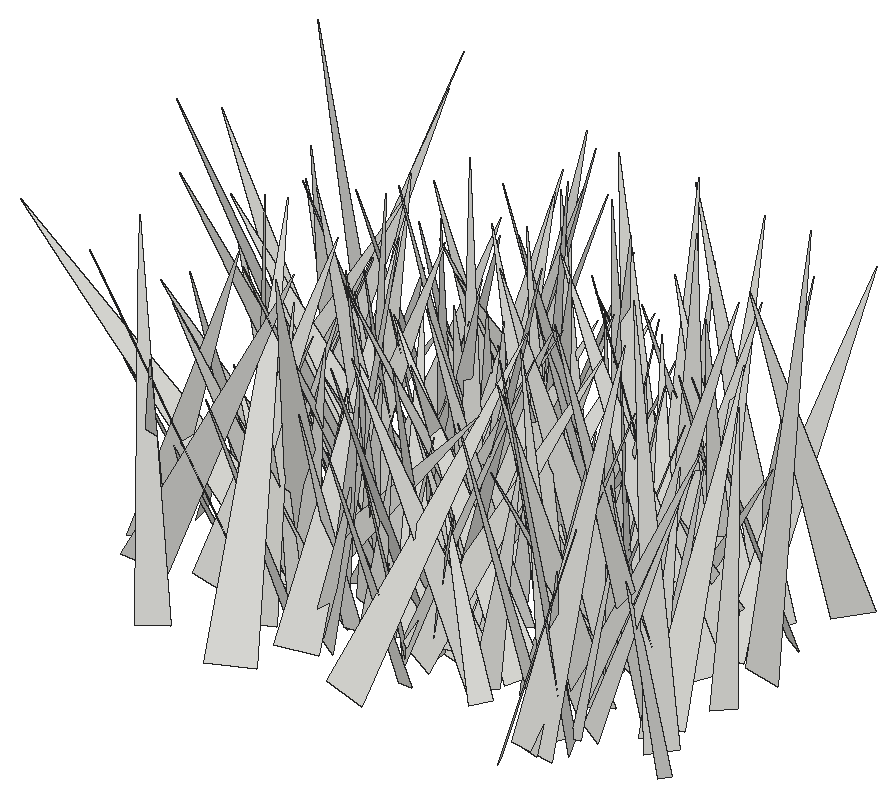
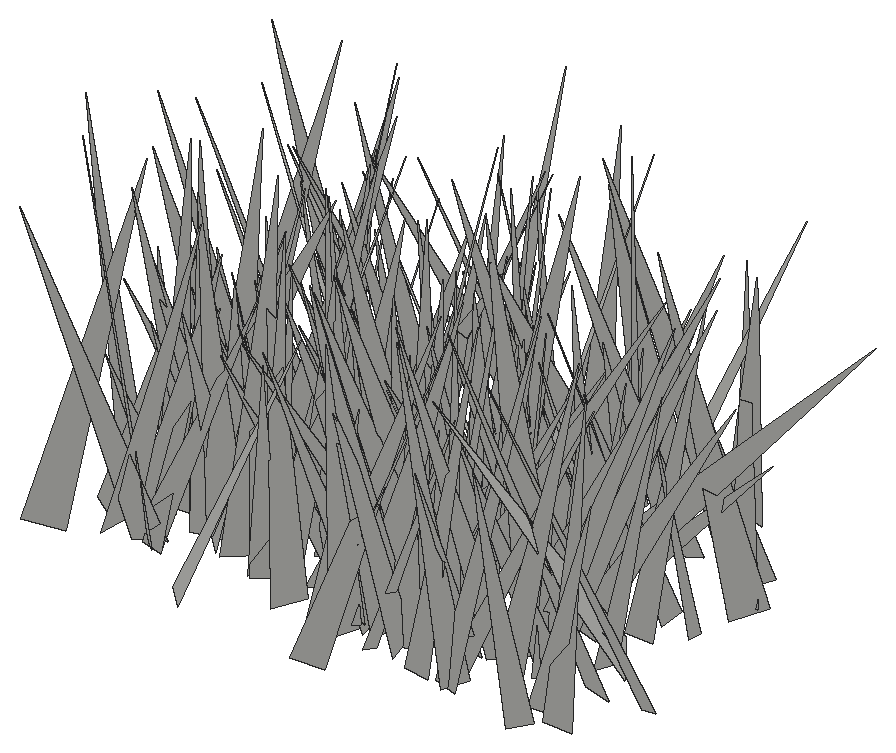
# SketchUp Ruby script. Lengths in inches.
U = 1.inch
M = Sketchup.active_model
def pt(a) = Geom::Point3d.new(a.map { |v| v * U })
def face(e, loops, mat)
  f = e.add_face(loops[0].map { |a| pt(a) })
  loops[1..].each { |l| e.add_face(l.map { |a| pt(a) }).erase! }
  f.material = f.back_material = mat if mat
  f
end
# faces: each face lists its corners as indices into pts; further lists are holes
def faces(e, pts, list, mat = nil) = list.each { |f| face(e, (f[0].is_a?(Array) ? f : [f]).map { |l| l.map { |i| pts[i] } }, mat) }
# xy, xz, yz: faces in a plane at the given z, y or x. An outline is a flat list of corners, or four numbers for a rectangle; further outlines are holes
def ring(l) = l.size == 4 ? [[l[0], l[1]], [l[2], l[1]], [l[2], l[3]], [l[0], l[3]]] : l.each_slice(2).to_a
def flat(e, list, mat, &to3) = list.each { |f| face(e, (f[0].is_a?(Array) ? f : [f]).map { |l| ring(l).map { |u, v| to3.(u, v) } }, mat) }
def xy(e, z, list, mat = nil) = flat(e, list, mat) { |x, y| [x, y, z] }
def xz(e, y, list, mat = nil) = flat(e, list, mat) { |x, z| [x, y, z] }
def yz(e, x, list, mat = nil) = flat(e, list, mat) { |y, z| [x, y, z] }
def lines(e, pts, list) = list.each { |a, b| e.add_line(pt(pts[a]), pt(pts[b])) }
# prism: a flat outline (further loops are holes) pulled along v
def prism(e, loops, v, mat = nil)
  f = face(e, loops, mat); d = Geom::Vector3d.new(v.map { |x| x * U })
  f.pushpull(f.normal.samedirection?(d) ? d.length : -d.length)
end
def box(e, o, s, mat = nil) = prism(e, [[o, [o[0] + s[0], o[1], o[2]], [o[0] + s[0], o[1] + s[1], o[2]], [o[0], o[1] + s[1], o[2]]]], [0, 0, s[2]], mat)
def at(x, y, z, deg = 0) = Geom::Transformation.translation(pt([x, y, z])) * Geom::Transformation.rotation(ORIGIN, Z_AXIS, deg.degrees)
def axes(o, x, y, z) = Geom::Transformation.new([*x, 0, *y, 0, *z, 0, *pt(o).to_a, 1])
def part(name) = M.definitions.add(name)
# library, detail: a bought-in or finely detailed component or shape, given as its bounding box
def library(name, o, s) = part(name).tap { |d| box(d.entities, o, s) }
def detail(e, o, s) = box(e.add_group.entities, o, s)
def put(e, d, t, mat = nil) = e.add_instance(d, t).tap { |i| i.material = mat if mat }
def group(e, t, mat = nil) = e.add_group.tap { |g| g.transformation = t; g.material = mat if mat }.entities
root = M.entities
c1 = part("fur_instance\#9")
p = [[0.8125,0,1.79],[0.67,-0.02,1.48],[0,-0.11,0],[0,0.11,0]]
faces(c1.entities,p,[[0,1,2,3]])
put(root,c1,axes([493.16,72.27,-21.86],[-2.05485,-3.90462,0.97999],[-3.96047,1.76344,-1.27819],[-0.72186,1.43981,4.22312]))
put(root,c1,axes([484.04,69.875,-21.66],[-0.66678,7.09806,0.59701],[6.83624,0.46921,2.05647],[-2.00116,-0.76214,6.82627]))
put(root,c1,axes([488.25,72.6,-21.86],[-2.14589,-4.13922,0.79032],[-4.13009,1.88974,-1.31675],[-0.83673,1.28775,4.4726]))
put(root,c1,axes([490.875,75.99,-21.86],[-2.64275,-7.72517,0.10148],[-7.35563,2.5487,2.46402],[2.36287,-0.70608,7.78402]))
put(root,c1,axes([485.3,73.87,-21.86],[-4.92734,-5.46841,0.2776],[-5.45988,4.87887,-0.80338],[-0.41255,0.74316,7.31688]))
put(root,c1,axes([500.3,72.47,-21.86],[-6.28358,-3.49392,1.76213],[-3.72095,6.36668,-0.64478],[1.21124,1.43309,7.16066]))
put(root,c1,axes([480.18,74.73,-21.86],[0.06322,-6.05576,0.15688],[-5.74231,-0.00994,1.93043],[1.92942,0.16885,5.74018]))
put(root,c1,axes([498.93,70.22,-21.86],[5.00084,3.55671,0.83126],[3.26277,-4.98345,1.69387],[-1.6418,0.92989,5.89825]))
put(root,c1,axes([487.64,69.6,-21.86],[-4.43994,6.98412,0.3729],[6.94517,4.45476,-0.74146],[0.82561,0.08476,8.24265]))
put(root,c1,axes([498.52,73.41,-21.86],[3.38817,-1.89067,0.4047],[-1.85762,-3.4096,-0.37677],[-0.53632,-0.13453,3.86165]))
put(root,c1,axes([499.5,71.25,-21.86],[1.47589,3.3854,0.35503],[3.34161,-1.51469,0.55196],[-0.64858,-0.1002,3.65165]))
put(root,c1,axes([499.47,71.32,-21.86],[0.16612,7.76506,1.97129],[7.95416,0.07536,-0.96713],[0.95574,-1.97685,7.70638]))
put(root,c1,axes([491.76,74.06,-21.86],[-3.13954,-2.86345,1.03549],[-2.74612,3.30524,0.81394],[1.31545,0.06589,4.17056]))
put(root,c1,axes([480.91,73.3,-21.86],[4.47531,-6.51665,1.20055],[-6.35255,-3.80729,3.0143],[1.88498,2.64087,7.30815]))
put(root,c1,axes([495.11,74.09,-21.86],[-6.35837,1.48,1.02188],[1.69793,6.17763,1.61781],[0.593,-1.81932,6.3247]))
put(root,c1,axes([488.86,72.93,-21.86],[3.38987,-1.12165,1.00676],[-1.27426,-3.45624,0.43994],[-0.80492,0.7478,3.54341]))
put(root,c1,axes([491.9,70.51,-21.86],[0.36828,7.38641,0.21711],[7.15433,-0.30198,-1.86176],[1.84979,-0.30261,7.15741]))
put(root,c1,axes([488.36,74.56,-21.86],[-1.36067,-5.7583,1.83351],[-5.61411,1.9,1.80082],[2.23642,1.26617,5.63617]))
put(root,c1,axes([495.96,72.91,-21.86],[-2.71204,2.5664,0.21286],[2.56651,2.66825,0.52947],[-0.21147,-0.53003,3.69611]))
put(root,c1,axes([499.19,75.12,-21.86],[1.49882,-6.76146,1.59023],[-6.75855,-1.79498,-1.262],[-1.60255,1.24632,6.80963]))
put(root,c1,axes([492.45,74.44,-21.86],[3.23905,1.92957,1.10614],[2.22288,-2.8741,-1.49551],[-0.07469,-1.85863,3.46094]))
put(root,c1,axes([490.24,74.02,-21.86],[2.26375,-3.28304,0.92587],[-3.40814,-2.22313,0.4499],[-0.14199,1.01955,3.96238]))
put(root,c1,axes([486.47,75.3,-21.66],[1.14957,-5.99203,1.40359],[-5.68779,-1.57972,-2.08556],[-2.35023,0.89221,5.73379]))
put(root,c1,axes([489.35,74.21,-21.86],[-0.77658,-4.10323,1.17838],[-4.23531,0.59015,-0.73621],[-0.53592,1.28194,4.11067]))
put(root,c1,axes([497.34,74.18,-21.86],[-4.90258,-2.23132,0.87524],[-2.28191,4.95484,-0.15015],[0.73329,0.50088,5.38438]))
put(root,c1,axes([499.65,72.49,-21.86],[-6.80477,1.06742,0.77743],[0.9228,6.76292,-1.20833],[0.94457,1.0827,6.78117]))
put(root,c1,axes([491.02,76.2,-21.66],[-2.08812,-6.42397,1.05341],[-6.15561,2.30841,1.87538],[2.11792,0.37569,6.48927]))
put(root,c1,axes([486.1,75.07,-21.86],[5.26826,5.58359,0.80335],[4.69893,-3.73546,-4.8521],[3.1212,-3.80083,5.9488]))
put(root,c1,axes([485.46,73.93,-21.86],[4.5767,5.68819,3.18986],[6.17982,-5.02762,0.09872],[-2.08339,-2.41752,7.30013]))
put(root,c1,axes([495.46,73.79,-21.86],[3.51253,-2.51047,1.78394],[-2.89575,-3.6135,0.61652],[-1.0486,1.56939,4.2732]))
put(root,c1,axes([485.29,77.09,-21.86],[6.31463,-5.10403,0.36931],[-4.97216,-6.25818,-1.47472],[-1.21044,-0.91981,7.98441]))
put(root,c1,axes([485.09,75.43,-21.86],[3.48904,-1.79502,0.75996],[-1.60226,-3.52839,-0.97792],[-1.11014,-0.54905,3.7999]))
put(root,c1,axes([504.12,72.79,-21.86],[-5.07583,-0.99149,0.0646],[-0.93064,4.62637,-2.11704],[-0.34804,2.08923,4.7186]))
put(root,c1,axes([490.82,74.28,-21.86],[2.69077,3.3772,1.27263],[3.60609,-2.57991,-0.77814],[-0.14558,-1.48455,4.24737]))
put(root,c1,axes([500.26,73.55,-21.86],[2.30047,4.4169,0.81433],[4.47004,-2.16262,-0.89782],[0.43686,-1.13065,4.89848]))
put(root,c1,axes([498.04,77.22,-21.86],[-4.51609,-3.87484,0.43498],[-3.47065,4.29803,2.25393],[1.77713,-1.453,5.5072]))
put(root,c1,axes([502,75.12,-21.66],[-1.47229,-7.46087,2.3597],[-7.72207,0.99683,-1.66627],[-1.2659,2.59656,7.41996]))
put(root,c1,axes([496.22,74.83,-21.66],[5.98331,3.57339,0.75673],[3.63565,-5.68637,-1.89446],[0.35186,-2.00943,6.70672]))
put(root,c1,axes([500.3,72.66,-21.66],[1.53322,3.39,0.04746],[3.12816,-1.43461,1.41479],[-1.30727,0.54307,3.44111]))
put(root,c1,axes([489.37,72.72,-21.86],[4.31579,6.0344,1.65644],[5.97789,-4.5707,1.07586],[-1.85004,-0.69181,7.34048]))
put(root,c1,axes([485.4,75.46,-21.86],[0.28978,-3.77503,0.68612],[-3.83038,-0.24462,0.27184],[0.22308,0.70349,3.77636]))
put(root,c1,axes([486.96,72.23,-21.66],[-5.33411,1.7362,0.45715],[1.45522,5.02033,-2.08679],[1.05153,1.85957,5.20696]))
put(root,c1,axes([498.81,74.43,-21.66],[3.86219,5.07234,0.99731],[5.04282,-3.42294,-2.11973],[1.1372,-2.04809,6.01264]))
put(root,c1,axes([490.53,74.68,-21.86],[5.38161,2.47127,3.67462],[2.66712,-6.4254,0.41515],[-3.53503,-1.08568,5.90733]))
put(root,c1,axes([483.8,73.36,-21.66],[-0.17372,7.00266,1.70424],[6.95108,0.61311,-1.81067],[1.90374,-1.5996,6.76675]))
put(root,c1,axes([484.52,74.32,-21.66],[-3.03964,-3.22245,0.08473],[-2.53096,2.3136,-2.80576],[-1.9964,1.97328,3.42802]))
put(root,c1,axes([479.75,74.93,-21.86],[5.60342,-3.67276,1.04707],[-3.81273,-5.48708,1.15708],[-0.22057,1.54484,6.59914]))
put(root,c1,axes([491.8,73.81,-21.86],[4.90909,4.36789,0.50992],[4.39704,-4.86378,-0.66882],[0.06695,-0.83837,6.53684]))
put(root,c1,axes([487.25,73.77,-21.86],[-4.58169,-0.00231,0.33908],[-0.10273,4.38765,-1.35823],[0.32316,1.36211,4.37574]))
put(root,c1,axes([485.61,75.91,-21.86],[-5.86481,5.71927,0.12396],[4.62698,4.63811,4.91939],[-3.36399,-3.59156,6.55024]))
put(root,c1,axes([487.5,78.6,-21.66],[-5.6893,-5.57398,0.54513],[-5.22917,5.56506,2.3282],[2.00554,-1.30211,7.61688]))
put(root,c1,axes([492.47,73.71,-21.66],[1.86343,6.88556,0.79652],[6.51007,-1.45535,-2.64927],[2.37997,-1.41024,6.62304]))
put(root,c1,axes([496.75,76.26,-21.86],[4.53456,1.85789,3.16607],[2.55783,-5.20835,-0.60709],[-2.63311,-1.85992,4.86266]))
put(root,c1,axes([485.8,75.9375,-21.86],[0.23103,-4.99246,1.62863],[-5.17408,0.0623,0.92493],[0.89778,1.64376,4.91147]))
put(root,c1,axes([488.94,71.58,-21.66],[-6.13074,4.86156,0.06985],[4.48302,5.69573,-2.94734],[1.88206,2.26926,7.24803]))
put(root,c1,axes([490.07,75.71,-21.66],[-2.15609,-3.98258,0.83043],[-3.73233,1.56246,-2.1972],[-1.61872,1.70208,3.96005]))
put(root,c1,axes([492.79,74.95,-21.86],[7.58691,1.58366,1.76713],[1.48707,-7.78642,0.59349],[-1.84915,0.23586,7.72768]))
put(root,c1,axes([496.28,74.88,-21.66],[-3.37764,5.82202,0.02709],[5.22944,3.02002,2.9728],[-2.55923,-1.51283,6.03878]))
put(root,c1,axes([485.65,75.42,-21.86],[-2.38468,3.13652,0.12042],[3.02513,2.25628,1.13874],[-0.83714,-0.7813,3.77197]))
put(root,c1,axes([493.81,78.08,-21.86],[-6.74137,-3.47517,0.05647],[-3.44773,6.70195,0.85032],[0.43951,-0.73012,7.53656]))
put(root,c1,axes([484.62,74.375,-21.86],[3.35621,4.76804,0.53975],[4.75729,-3.3924,0.38655],[-0.62744,-0.21695,5.81798]))
put(root,c1,axes([503.14,73.84,-21.66],[-7.7657,1.30292,0.44128],[1.14319,7.51969,-2.08465],[0.76515,1.98873,7.59328]))
put(root,c1,axes([492.96,74.78,-21.86],[0.42201,3.83383,0.13948],[3.79822,-0.3978,-0.55775],[0.53966,-0.19825,3.81644]))
put(root,c1,axes([486.6,74.625,-21.86],[3.67967,2.76321,1.03507],[2.46473,-3.78797,1.35021],[-1.62229,0.51247,4.39911]))
put(root,c1,axes([495.53,77.25,-21.86],[-0.9776,-5.25666,1.94415],[-5.10339,1.65068,1.89699],[2.31681,1.41798,4.99896]))
put(root,c1,axes([493.32,74.91,-21.66],[-2.78361,3.37072,1.19614],[3.02117,3.0272,-1.49988],[1.91443,0.12385,4.10617]))
put(root,c1,axes([502.02,74.66,-21.86],[-4.30895,1.90574,0.59057],[1.67064,4.21479,-1.41144],[1.09067,1.07302,4.49519]))
put(root,c1,axes([490.04,77.36,-21.86],[-0.65259,-3.58567,0.77528],[-3.62638,0.74954,0.41412],[0.55447,0.682,3.62097]))
put(root,c1,axes([481.67,78.54,-21.86],[-0.57876,-6.04691,0.53315],[-6.05695,0.61084,0.35302],[0.40347,0.49606,6.06428]))
put(root,c1,axes([489.11,77.16,-21.66],[1.07794,-7.21694,3.00432],[-7.53412,-1.768,-1.54384],[-2.08502,2.65746,7.13181]))
put(root,c1,axes([491.26,74.95,-21.86],[-1.93628,5.55,0.46539],[5.55779,1.89356,0.54185],[-0.36056,-0.61659,5.85304]))
put(root,c1,axes([488.66,75.8,-21.86],[3.17531,6.56755,2.54139],[6.79761,-3.58673,0.77578],[-1.83954,-1.91744,7.25351]))
put(root,c1,axes([487.5625,78.01,-21.86],[2.55514,-3.36467,0.69917],[-3.31318,-2.64324,-0.61213],[-0.91251,0.1757,4.18031]))
put(root,c1,axes([486.22,76.21,-21.66],[3.6811,-6.05089,2.6185],[-6.53456,-2.94932,2.37094],[0.87715,3.42178,6.67401]))
put(root,c1,axes([492.45,77.01,-21.86],[-3.8674,0.14725,0.40736],[0.1724,3.88071,0.23399],[0.39736,-0.25058,3.86312]))
put(root,c1,axes([497.97,74.56,-21.86],[-8.22184,1.12863,0.67504],[0.91948,7.98903,-2.15825],[0.94024,2.05661,8.01339]))
put(root,c1,axes([480.26,77.26,-21.86],[3.62066,0.28745,0.41277],[0.34104,-3.60783,-0.479],[-0.36973,-0.51296,3.60033]))
put(root,c1,axes([493.85,77.6,-21.66],[-0.12405,-5.8754,2.10648],[-6.00776,-0.4589,-1.63376],[-1.69244,2.05962,5.64504]))
put(root,c1,axes([487.54,79.42,-21.66],[-3.32814,-6.39102,1.50803],[-6.07577,3.63841,2.01068],[2.49085,0.3356,6.91945]))
put(root,c1,axes([487.49,76.84,-21.86],[4.11337,-1.35782,0.42666],[-1.42017,-4.00175,0.95638],[-0.09392,1.04301,4.22479]))
put(root,c1,axes([487.9,77.13,-21.86],[-3.35833,-3.2337,1.73378],[-3.57177,3.41915,-0.54142],[0.83981,1.61055,4.63056]))
put(root,c1,axes([490.22,80.32,-21.66],[5.08436,-3.96797,0.13679],[-3.71243,-4.83007,-2.12193],[-1.40762,-1.5937,6.0904]))
put(root,c1,axes([481.64,76.8,-21.86],[4.44559,-0.41699,0.42413],[-0.48383,-4.39553,0.74982],[-0.34594,0.78895,4.4017]))
put(root,c1,axes([497.54,78.56,-21.66],[2.58278,-6.81445,2.81399],[-6.72051,-3.40212,-2.07037],[-3.03151,1.73634,6.98721]))
put(root,c1,axes([502.14,75.22,-21.66],[-4.09876,5.0884,1.14662],[4.86258,4.25523,-1.50159],[1.8873,0.0873,6.359]))
put(root,c1,axes([488.97,77.59,-21.86],[-5.40914,1.11965,1.3835],[1.23539,5.5484,0.3398],[1.28121,-0.62292,5.51334]))
put(root,c1,axes([483.52,79.38,-21.86],[0.83306,-5.07313,1.39633],[-4.3947,-1.44829,-2.63999],[-2.89363,0.73905,4.41148]))
put(root,c1,axes([495.43,79.36,-21.86],[1.75124,-3.26229,0.83742],[-3.12175,-1.92651,-0.97669],[-1.26432,0.23809,3.57148]))
put(root,c1,axes([488.97,79.05,-21.86],[2.93254,-6.52755,1.0505],[-6.19008,-2.30697,2.94501],[2.32281,2.09313,6.52193]))
put(root,c1,axes([488.57,79.72,-21.86],[-0.29394,-4.28793,0.2812],[-4.0742,0.18848,-1.38464],[-1.36614,0.36048,4.06885]))
put(root,c1,axes([488.78,80.11,-21.86],[-3.34858,-4.98605,1.16696],[-4.83329,3.53804,1.24784],[1.69169,0.23891,5.87509]))
put(root,c1,axes([491.71,79.5,-21.86],[-7.3935,-3.44968,1.78048],[-3.41196,7.60131,0.55924],[1.85173,0.23234,8.13949]))
put(root,c1,axes([500.63,76.88,-21.66],[-3.9364,0.91485,1.26316],[0.41585,3.92071,-1.54367],[1.50319,1.31107,3.73488]))
put(root,c1,axes([493.23,80.95,-21.66],[5.19652,-2.78136,0.42044],[-2.54268,-5.02221,-1.79688],[-1.20313,-1.39929,5.61347]))
put(root,c1,axes([498.26,77.73,-21.66],[2.40948,7.1196,1.80641],[7.28749,-2.07931,-1.52526],[0.91887,-2.17835,7.35989]))
put(root,c1,axes([488.34,79.875,-21.86],[-7.10232,2.48969,0.17848],[2.39972,6.66255,2.55443],[-0.68683,-2.46683,7.07929]))
put(root,c1,axes([484.66,79.36,-21.86],[1.69765,-3.69471,0.41656],[-3.54176,-1.46758,1.41724],[1.13153,0.9496,3.81108]))
put(root,c1,axes([492.5,76.81,-21.86],[1.13757,8.04859,1.54719],[7.76789,-1.55698,2.3882],[-2.61411,-1.12413,7.76984]))
put(root,c1,axes([489.38,77.33,-21.86],[-2.89965,3.32427,1.06428],[2.78447,3.03733,-1.90073],[2.1048,0.5615,3.98069]))
put(root,c1,axes([502.71,77.75,-21.86],[-4.9436,1.78617,0.77223],[1.56135,4.89918,-1.33648],[1.16143,1.01666,5.08364]))
put(root,c1,axes([501.0625,78.72,-21.66],[-3.57057,6.8988,1.02898],[6.50769,2.8788,3.28081],[-2.51043,-2.34953,7.04122]))
put(root,c1,axes([483.25,81.69,-21.66],[0.03934,-7.1777,0.79174],[-6.87762,-0.27857,-2.18369],[-2.20103,0.74216,6.83757]))
put(root,c1,axes([498.2,77.43,-21.86],[-6.18556,-0.57175,1.0735],[-0.94708,5.75521,-2.39186],[0.76312,2.5082,5.73298]))
put(root,c1,axes([484.83,80.61,-21.66],[-3.02685,-7.70536,1.30124],[-7.48247,2.45538,-2.86554],[-2.25353,2.19686,7.76679]))
put(root,c1,axes([496.55,80.3,-21.86],[-4.3896,-2.50757,2.34029],[-2.3133,4.97071,0.98703],[2.5325,0.19407,4.95805]))
put(root,c1,axes([494.53,79.03,-21.86],[-6.29408,3.56033,1.19684],[3.6784,6.31519,0.55815],[0.76008,-1.07993,7.20971]))
put(root,c1,axes([495.375,79.7,-21.86],[0.04539,-4.24616,1.86431],[-4.44886,0.48634,1.21602],[1.30888,1.80033,4.06857]))
put(root,c1,axes([487.52,79.37,-21.86],[5.08569,0.11573,0.95874],[0.07501,-5.17107,0.22632],[-0.96278,0.20845,5.08197]))
put(root,c1,axes([485.05,79.7,-21.86],[-2.73382,6.12597,3.74599],[6.6709,3.64992,-1.10045],[2.6569,-2.86083,6.61742]))
put(root,c1,axes([488.39,81.15,-21.86],[-3.41179,-1.77285,0.16017],[-1.67154,3.30984,1.02951],[0.61205,-0.84317,3.70451]))
put(root,c1,axes([487.1,81.73,-21.66],[1.41766,-6.83451,0.48866],[-6.53171,-1.19719,2.20513],[2.07029,0.90294,6.62252]))
put(root,c1,axes([487.97,79.57,-21.66],[4.83025,3.81866,0.07193],[3.65702,-4.5907,-1.86288],[1.10161,-1.50398,5.86882]))
put(root,c1,axes([489.02,81.15,-21.86],[3.24454,-4.71501,1.03025],[-4.7617,-3.32972,-0.24278],[-0.78672,0.70811,5.71834]))
put(root,c1,axes([481.32,80.81,-21.86],[-5.12264,0.34016,1.65759],[0.60899,5.30124,0.79415],[1.57874,-0.94118,5.07212]))
put(root,c1,axes([496.36,78.82,-21.86],[3.89284,1.77366,0.49192],[1.64576,-3.86945,0.92782],[-0.82421,0.65077,4.17603]))
put(root,c1,axes([496.83,79.75,-21.86],[-7.44301,-3.63877,0.95843],[-3.76282,7.20814,-1.85509],[0.01898,2.08796,8.0745]))
put(root,c1,axes([490.09,80.75,-21.86],[4.42383,-2.92058,1.2942],[-2.99041,-4.56361,-0.07677],[-1.12348,0.64702,5.30039]))
put(root,c1,axes([492.28,79.63,-21.86],[-1.46329,-3.87448,2.4887],[-4.52721,1.6881,-0.03379],[0.84239,2.34204,4.14146]))
put(root,c1,axes([500.63,82.02,-21.86],[2.63611,-2.6678,0.56163],[-2.26437,-2.5776,-1.61563],[-1.51829,-0.78771,3.38467]))
put(root,c1,axes([498.41,79.66,-21.66],[4.05513,-1.76427,0.28786],[-1.75227,-3.78191,1.50543],[0.35366,1.49134,4.15818]))
put(root,c1,axes([491.34,78.47,-21.86],[-5.55671,4.70477,2.20019],[4.40361,5.97611,-1.65743],[2.7539,-0.06297,7.08977]))
put(root,c1,axes([495.97,80,-21.86],[4.05853,2.67005,1.15678],[2.78357,-4.14094,-0.20805],[-0.84796,-0.81387,4.85361]))
put(root,c1,axes([499.875,81.37,-21.86],[0.14601,-6.62439,2.10053],[-6.94709,-0.08453,0.21629],[0.18059,2.1039,6.62247]))
put(root,c1,axes([498.88,79.24,-21.86],[-4.29612,3.71614,0.38084],[3.69784,4.31285,-0.36964],[0.52979,0.03157,5.66831]))
put(root,c1,axes([493.76,83.04,-21.86],[-1.16201,-7.65185,1.0654],[-7.72512,1.16361,-0.06847],[0.09162,1.06366,7.73928]))
put(root,c1,axes([483.62,81.5,-21.86],[-7.37091,1.53228,0.84327],[1.65266,7.29739,1.18581],[0.57246,-1.33774,7.43452]))
put(root,c1,axes([497.25,82.38,-21.86],[-4.80805,-4.95386,1.3489],[-5.02147,4.92244,0.17909],[1.0701,0.84054,6.90116]))
put(root,c1,axes([499.9,81.78,-21.86],[1.52237,-3.55739,1.37163],[-3.65271,-1.78416,-0.57315],[-1.09275,1.00785,3.82677]))
put(root,c1,axes([491.27,80.42,-21.66],[5.10289,-1.83511,1.25864],[-2.13691,-4.91957,1.49087],[-0.62081,1.84972,5.21387]))
put(root,c1,axes([495.57,79.15,-21.86],[-7.58228,1.17889,0.51367],[1.00041,7.33787,-2.07353],[0.80796,1.97752,7.38791]))
put(root,c1,axes([482.33,83.2,-21.66],[3.64505,-0.39812,0.27738],[-0.20845,-3.18305,-1.82936],[-0.43816,-1.79764,3.17779]))
put(root,c1,axes([489.04,80.33,-21.66],[-0.29614,5.30233,1.4786],[4.87042,0.94241,-2.40408],[2.56516,-1.17721,4.73528]))
put(root,c1,axes([495.72,79.21,-21.86],[3.73526,4.02595,0.93613],[3.5763,-3.78049,1.98866],[-2.07237,0.73241,5.11915]))
put(root,c1,axes([501.71,82.78,-21.86],[-3.13069,-4.74867,0.6646],[-4.79451,3.11096,-0.35688],[0.06511,0.75154,5.67659]))
put(root,c1,axes([499.71,79.76,-21.86],[-0.4926,4.67354,0.05511],[4.67276,0.49124,0.10792],[-0.10156,-0.0661,4.69819]))
put(root,c1,axes([502.33,80.3125,-21.86],[2.12447,7.8086,2.15105],[8.03257,-2.31646,0.47574],[-1.03873,-1.94278,8.07844]))
put(root,c1,axes([489.92,84.34,-21.66],[-0.39765,-7.51588,0.89638],[-7.02687,0.7002,2.75371],[2.81337,0.68655,7.00455]))
put(root,c1,axes([486.05,83.36,-21.66],[6.38697,0.74513,2.00431],[1.2691,-6.40204,-1.66407],[-1.72101,-1.95564,6.21124]))
put(root,c1,axes([491.24,79.65,-21.86],[-0.72981,5.66267,0.18679],[5.27184,0.7477,-2.06932],[2.0757,0.09199,5.32132]))
put(root,c1,axes([487.55,83.36,-21.86],[-0.07367,-4.26522,0.50041],[-4.16979,0.19077,1.01214],[1.02732,0.46845,4.14405]))
put(root,c1,axes([497.49,82.14,-21.86],[1.282,-6.99581,3.06835],[-7.6361,-1.26107,0.31524],[-0.21483,3.07701,7.10532]))
put(root,c1,axes([500.6,78.99,-21.66],[0.70826,8.01559,0.32411],[7.89046,-0.75477,1.42384],[-1.44754,-0.19233,7.91985]))
put(root,c1,axes([489.875,79.69,-21.66],[7.02888,1.27959,1.54515],[0.73768,-6.88381,2.34499],[-1.86566,2.099,6.7486]))
put(root,c1,axes([497.12,81.0625,-21.86],[0.03903,6.40601,1.64221],[6.43648,0.34027,-1.48032],[1.51842,-1.60705,6.23275]))
put(root,c1,axes([491.02,82.33,-21.86],[7.15031,1.42356,2.57616],[1.59453,-7.56218,-0.24693],[-2.47399,-0.75958,7.28646]))
put(root,c1,axes([500.76,80.6,-21.86],[-1.96871,3.37657,0.07437],[3.27614,1.93014,-0.90775],[0.82077,0.39482,3.80171]))
put(root,c1,axes([493.3,80.75,-21.86],[4.64309,0.99306,0.50279],[0.80416,-4.48393,1.43003],[-0.7696,1.30595,4.52764]))
put(root,c1,axes([492.46,82.62,-21.86],[-3.73947,1.85603,0.44676],[1.90802,3.6015,1.00834],[-0.06253,-1.10111,4.05114]))
put(root,c1,axes([481.875,82.875,-21.66],[2.63596,-3.80697,0.02165],[-3.40971,-2.34911,2.07299],[1.69332,1.196,4.14053]))
put(root,c1,axes([488.19,83.46,-21.86],[4.14097,0.37336,0.37849],[0.46882,-3.96604,-1.21698],[-0.25072,-1.24957,3.97567]))
put(root,c1,axes([498.63,84.01,-21.86],[-1.84979,-4.95748,0.73449],[-4.97918,1.90688,0.3307],[0.56907,0.57009,5.281]))
put(root,c1,axes([487.7,83.43,-21.86],[0.8315,-3.67241,0.7269],[-3.73531,-0.86356,-0.09004],[-0.24991,0.6885,3.76429]))
put(root,c1,axes([488.5,80.65,-21.66],[6.0321,-2.57805,3.10449],[-3.62742,-5.91038,2.14001],[-1.76807,3.33038,6.20104]))
put(root,c1,axes([487.375,84.01,-21.86],[0.2797,-5.08952,0.70223],[-5.01624,-0.11848,1.13926],[1.11073,0.74654,4.96825]))
put(root,c1,axes([500.15,82.15,-21.86],[-4.76226,4.46867,0.77555],[4.53262,4.64929,1.04363],[-0.16086,-1.29026,6.44663]))
put(root,c1,axes([485.49,83.37,-21.86],[-3.66042,-4.84933,0.70173],[-4.78346,3.34689,-1.82316],[-1.06154,1.63996,5.79575]))
put(root,c1,axes([489.51,83.56,-21.66],[0.21483,-6.37799,2.26736],[-6.52313,-0.80094,-1.63496],[-1.80789,2.13204,6.16862]))
put(root,c1,axes([494.8,82.29,-21.86],[-6.8831,0.44539,2.18741],[0.27023,7.20464,-0.61666],[2.21588,0.50489,6.86987]))
put(root,c1,axes([484.42,82.59,-21.86],[1.25839,-5.65908,2.69216],[-6.0262,-0.33916,2.10388],[1.71982,2.95233,5.40207]))
put(root,c1,axes([495.78,82.43,-21.86],[-6.05615,5.17907,2.30301],[5.46239,6.23254,0.34836],[1.51293,-1.77094,7.96105]))
put(root,c1,axes([494.36,83.27,-21.86],[2.05705,-3.40779,1.21765],[-3.60141,-2.06493,0.30505],[-0.3543,1.20424,3.9688]))
put(root,c1,axes([484.75,85.3,-21.86],[-2.90954,-6.16313,0.64564],[-6.10361,2.97343,0.8781],[1.07095,0.20243,6.75859]))
put(root,c1,axes([478.22,82.34,-21.86],[3.46284,5.45761,0.55951],[5.19477,-3.049,-2.40992],[1.76435,-1.73432,5.99742]))
put(root,c1,axes([488.29,81.5,-21.66],[6.56769,-0.93589,1.93904],[-1.50422,-6.44796,1.98276],[-1.54048,2.30611,6.3308]))
put(root,c1,axes([490.3,85.27,-21.86],[-5.70608,-2.81682,0.48614],[-2.67601,5.6456,1.30244],[1.0049,-0.96065,6.22877]))
put(root,c1,axes([488.42,84.84,-21.86],[-4.22859,-0.79072,0.99748],[-0.41595,4.12901,1.5098],[1.20299,-1.35177,4.02824]))
put(root,c1,axes([486.1,85.2,-21.86],[-1.823,-5.96341,0.88128],[-5.94354,1.93183,0.77754],[1.00658,0.60664,6.18716]))
put(root,c1,axes([492.53,84.12,-21.86],[6.63287,-1.89646,1.66739],[-1.83678,-6.83922,-0.47211],[-1.73291,-0.0097,6.88248]))
put(root,c1,axes([498.01,80.46,-21.86],[-6.32088,1.55628,0.92222],[1.03646,5.86264,-2.78949],[1.48264,2.53644,5.88169]))
put(root,c1,axes([499.07,83.5625,-21.86],[-1.92463,-5.23066,1.71698],[-5.26178,1.21283,-2.20335],[-1.6191,2.27625,5.1195]))
put(root,c1,axes([496.85,82.03,-21.86],[-1.18605,7.62635,1.82441],[7.84154,1.15487,0.27022],[0.00582,-1.84431,7.7133]))
put(root,c1,axes([498.67,84.1,-21.66],[5.37674,4.78999,2.15375],[5.23773,-5.117,-1.69543],[-0.38579,-2.71372,6.99849]))
put(root,c1,axes([502.29,85.37,-21.66],[3.31279,-6.01066,2.01721],[-5.81791,-3.7865,-1.72802],[-2.51972,0.84034,6.64203]))
put(root,c1,axes([489.21,87.27,-21.66],[4.98513,-4.06782,0.78587],[-3.3159,-4.65458,-3.05875],[-2.48386,-1.95039,5.66063]))
put(root,c1,axes([485.5,82.85,-21.86],[0.89706,4.01856,0.51185],[4.05094,-0.89322,-0.08685],[-0.02607,-0.51851,4.11655]))
put(root,c1,axes([484.54,85.03,-21.86],[6.03259,-1.06555,0.38284],[-1.02373,-6.01977,-0.62323],[-0.48366,-0.54868,6.09418]))
put(root,c1,axes([494.69,82.85,-21.86],[-4.5808,2.50643,0.71678],[2.42315,4.62824,-0.69815],[0.96142,0.27723,5.1748]))
put(root,c1,axes([479.98,85.15,-21.86],[-0.39451,-5.89979,1.57703],[-6.09619,0.47415,0.24879],[0.36204,1.55494,5.90773]))
put(root,c1,axes([480.38,82.47,-21.86],[3.15625,6.97995,0.87784],[7.00121,-3.02246,-1.14023],[0.68808,-1.26383,7.57506]))
put(root,c1,axes([500.6,83.29,-21.86],[-7.87651,1.28049,0.44694],[1.23259,7.85729,-0.78901],[0.56579,0.70864,7.94081]))
put(root,c1,axes([481.15,79.95,-21.86],[6.66219,5.05954,0.23915],[4.47229,-6.06129,3.64695],[-2.37798,2.77537,7.52884]))
put(root,c1,axes([483.51,83.39,-21.66],[1.68916,7.29229,2.94864],[7.0223,-2.75681,2.79508],[-3.5439,-1.98689,6.94394]))
put(root,c1,axes([490.73,84.65,-21.86],[-2.55012,3.64542,1.48438],[3.93085,2.44958,0.73729],[0.20222,-1.64502,4.38733]))
put(root,c1,axes([489.4,83.48,-21.86],[5.64038,0.84844,0.8162],[0.68974,-5.61874,1.07421],[-0.95409,0.95384,5.60177]))
put(root,c1,axes([481.07,84.59,-21.86],[-2.03282,4.17049,1.29504],[4.34211,1.77825,1.08919],[-0.46493,-1.62705,4.50988]))
put(root,c1,axes([488.66,83.31,-21.86],[6.53232,-2.04401,3.08815],[-2.89411,-6.72439,1.67109],[-2.31057,2.64395,6.63752]))
put(root,c1,axes([495.87,86.18,-21.86],[-3.87501,-4.05549,0.17386],[-4.05477,3.85598,-0.42797],[-0.18982,0.42113,5.59281]))
put(root,c1,axes([487.625,84.06,-21.86],[6.99973,1.86447,1.44835],[1.77883,-7.14461,0.6004],[-1.55233,0.22015,7.21886]))
put(root,c1,axes([481.04,85.87,-21.86],[3.52002,-2.83902,0.00242],[-2.82378,-3.50072,0.47096],[0.29379,0.3681,4.49764]))
put(root,c1,axes([499.02,83.63,-21.86],[0.16958,6.97336,1.46095],[6.91324,0.19239,-1.72074],[1.72314,-1.45812,6.75984]))
put(root,c1,axes([489.71,84.47,-21.86],[4.97353,-2.18793,2.98402],[-2.79783,-5.49524,0.634],[-2.42149,1.85546,5.39639]))
